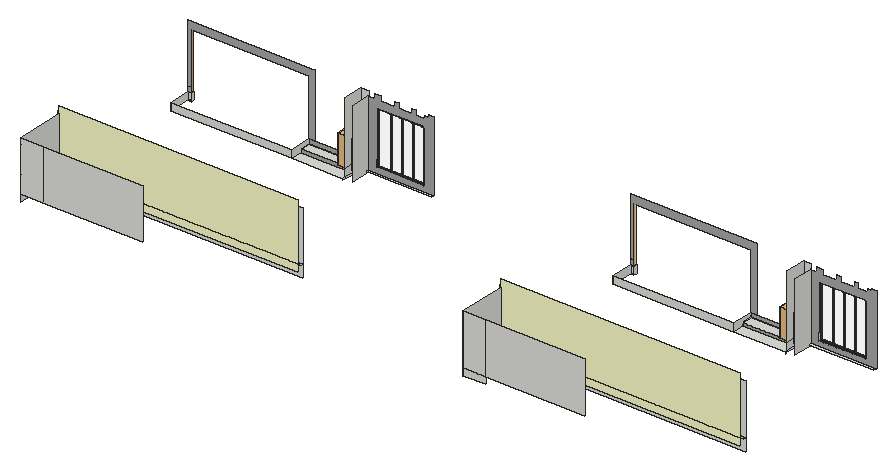
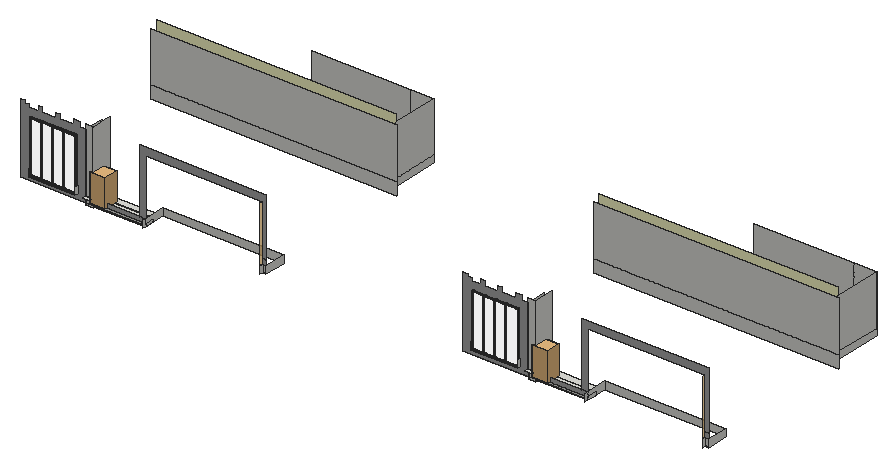
# SketchUp Ruby script. Lengths in inches.
U = 1.inch
M = Sketchup.active_model
def pt(a) = Geom::Point3d.new(a.map { |v| v * U })
def face(e, loops, mat)
  f = e.add_face(loops[0].map { |a| pt(a) })
  loops[1..].each { |l| e.add_face(l.map { |a| pt(a) }).erase! }
  f.material = f.back_material = mat if mat
  f
end
# faces: each face lists its corners as indices into pts; further lists are holes
def faces(e, pts, list, mat = nil) = list.each { |f| face(e, (f[0].is_a?(Array) ? f : [f]).map { |l| l.map { |i| pts[i] } }, mat) }
# xy, xz, yz: faces in a plane at the given z, y or x. An outline is a flat list of corners, or four numbers for a rectangle; further outlines are holes
def ring(l) = l.size == 4 ? [[l[0], l[1]], [l[2], l[1]], [l[2], l[3]], [l[0], l[3]]] : l.each_slice(2).to_a
def flat(e, list, mat, &to3) = list.each { |f| face(e, (f[0].is_a?(Array) ? f : [f]).map { |l| ring(l).map { |u, v| to3.(u, v) } }, mat) }
def xy(e, z, list, mat = nil) = flat(e, list, mat) { |x, y| [x, y, z] }
def xz(e, y, list, mat = nil) = flat(e, list, mat) { |x, z| [x, y, z] }
def yz(e, x, list, mat = nil) = flat(e, list, mat) { |y, z| [x, y, z] }
def lines(e, pts, list) = list.each { |a, b| e.add_line(pt(pts[a]), pt(pts[b])) }
# prism: a flat outline (further loops are holes) pulled along v
def prism(e, loops, v, mat = nil)
  f = face(e, loops, mat); d = Geom::Vector3d.new(v.map { |x| x * U })
  f.pushpull(f.normal.samedirection?(d) ? d.length : -d.length)
end
def box(e, o, s, mat = nil) = prism(e, [[o, [o[0] + s[0], o[1], o[2]], [o[0] + s[0], o[1] + s[1], o[2]], [o[0], o[1] + s[1], o[2]]]], [0, 0, s[2]], mat)
def at(x, y, z, deg = 0) = Geom::Transformation.translation(pt([x, y, z])) * Geom::Transformation.rotation(ORIGIN, Z_AXIS, deg.degrees)
def axes(o, x, y, z) = Geom::Transformation.new([*x, 0, *y, 0, *z, 0, *pt(o).to_a, 1])
def part(name) = M.definitions.add(name)
# library, detail: a bought-in or finely detailed component or shape, given as its bounding box
def library(name, o, s) = part(name).tap { |d| box(d.entities, o, s) }
def detail(e, o, s) = box(e.add_group.entities, o, s)
def put(e, d, t, mat = nil) = e.add_instance(d, t).tap { |i| i.material = mat if mat }
def group(e, t, mat = nil) = e.add_group.tap { |g| g.transformation = t; g.material = mat if mat }.entities
root = M.entities
M.materials.add("Glazing").color = [128, 128, 128]
M.materials["Glazing"].alpha = 0.05
M.materials.add("Powdercoating").color = [41, 44, 40]
M.materials.add("[Color E01]").color = [255, 255, 204]
M.materials.add("[Color M03]1").color = [170, 170, 170]
M.materials.add("[Wood OSB]").color = [255, 207, 129]
M.materials["[Wood OSB]"].alpha = 0.8
c1 = library("plant1",[-367.84,-375.82,-125.45],[750.59,696.16,1346.74])
c2 = part("skp4FF")
put(c2.entities,c1,at(0,0,0))
c3 = part("Group\#15")
xy(c3.entities,0,[[0,-55.94,0.71,45.94]])
xy(c3.entities,0.2,[[0,-55.94,0.47,45.94],[0.47,45.94,0.71,46.42]])
xy(c3.entities,2.36,[[0.47,-55.94,0.71,46.42]])
xz(c3.entities,-55.94,[[0,0,0.71,0,0.71,2.36,0.47,2.36,0.47,0.2,0,0.2]])
xz(c3.entities,45.94,[[0,0,0.71,0.2]])
xz(c3.entities,46.42,[[0.47,0.2,0.71,2.36]])
yz(c3.entities,0,[[-55.94,0,45.94,0.2]])
yz(c3.entities,0.47,[[-55.94,0.2,46.42,2.36]])
yz(c3.entities,0.71,[[-55.94,0,45.94,0,45.94,0.2,46.42,0.2,46.42,2.36,-55.94,2.36]])
c4 = part("Group\#7")
xy(c4.entities,0,[[0,-59.09,0.71,45.94]])
xy(c4.entities,0.2,[[0,-59.09,0.47,45.94],[0.47,45.94,0.71,46.42]])
xy(c4.entities,2.36,[[0.47,-59.09,0.71,46.42]])
xz(c4.entities,-59.09,[[0,0,0.71,0,0.71,2.36,0.47,2.36,0.47,0.2,0,0.2]])
xz(c4.entities,45.94,[[0,0,0.71,0.2]])
xz(c4.entities,46.42,[[0.47,0.2,0.71,2.36]])
yz(c4.entities,0,[[-59.09,0,45.94,0.2]])
yz(c4.entities,0.47,[[-59.09,0.2,46.42,2.36]])
yz(c4.entities,0.71,[[-59.09,0,45.94,0,45.94,0.2,46.42,0.2,46.42,2.36,-59.09,2.36]])
c5 = part("Group\#16")
prism(c5.entities,[[[0.47,-56.18,0.2],[0,-56.18,0.2],[0,-56.18,0],[0.71,-56.18,0],[0.71,-56.18,2.36],[0.47,-56.18,2.36]]],[0,28.68,0])
c6 = part("Group\#10")
box(c6.entities,[-0.73,0,0],[27.99,0.55,102.05])
c7 = part("Group\#18")
xy(c7.entities,0,[[0.47,-56.18,0.47,-55.47,0,-55.47,0,-28.21,1.18,-28.21,1.18,-56.18]])
xy(c7.entities,0.2,[[0.71,-56.18,1.18,-28.21],[0,-55.47,0.47,-28.21],[0.47,-28.21,0.71,-27.74]])
xy(c7.entities,2.36,[[0.47,-56.18,0.71,-27.74]])
xz(c7.entities,-56.18,[[0.47,0,1.18,0,1.18,0.2,0.71,0.2,0.71,2.36,0.47,2.36]])
xz(c7.entities,-55.47,[[0,0,0.47,0.2]])
xz(c7.entities,-28.21,[[0,0,1.18,0.2]])
xz(c7.entities,-27.74,[[0.47,0.2,0.71,2.36]])
yz(c7.entities,0,[[-55.47,0,-28.21,0.2]])
yz(c7.entities,0.47,[[-56.18,0,-55.47,0.2],[-56.18,0.2,-27.74,2.36]])
yz(c7.entities,0.71,[[-56.18,0.2,-27.74,2.36]])
yz(c7.entities,1.18,[[-56.18,0,-28.21,0.2]])
c8 = part("Group\#34")
xy(c8.entities,0,[[-20.45,0,7.76,1.22]])
xy(c8.entities,0.06,[[-20.39,0.06,7.7,1.22]])
xy(c8.entities,0.47,[[-19.98,0,7.28,0.06]])
xy(c8.entities,101.89,[[-19.98,0,7.28,0.06]])
xy(c8.entities,102.3,[[-20.39,0.06,7.7,1.22]])
xy(c8.entities,102.36,[[-20.45,0,7.76,1.22]])
xz(c8.entities,0,[[[-20.45,0,7.76,102.36],[-19.98,0.47,7.28,101.89]]])
xz(c8.entities,0.06,[[[-20.39,0.06,7.7,102.3],[-19.98,0.47,7.28,101.89]]])
xz(c8.entities,1.22,[[[-20.45,0,7.76,102.36],[-20.39,0.06,7.7,102.3]]])
yz(c8.entities,-20.45,[[0,0,1.22,102.36]])
yz(c8.entities,-20.39,[[0.06,0.06,1.22,102.3]])
yz(c8.entities,-19.98,[[0,0.47,0.06,101.89]])
yz(c8.entities,7.28,[[0,0.47,0.06,101.89]])
yz(c8.entities,7.7,[[0.06,0.06,1.22,102.3]])
yz(c8.entities,7.76,[[0,0,1.22,102.36]])
c9 = part("Group\#6")
put(c9.entities,c3,axes([27.97,0,7.875],[1,0,0],[0,0,-1],[0,1,0]),"Powdercoating")
put(c9.entities,c4,axes([0.71,0,6.8],[-1,0,0],[0,0,-0.97687],[0,1,0]),"Powdercoating")
put(c9.entities,c5,axes([-27.5,0,-38.07],[0,0,-1],[-1,0,0],[0,1,0]),"Powdercoating")
put(c9.entities,c6,at(1.12,0.35,-38.39),"Glazing")
put(c9.entities,c7,axes([-27.5,0,63.35],[0,0,1],[-1,0,0],[0,1,0]),"Powdercoating")
put(c9.entities,c8,at(20.6875,1.0625,-38.54),"Powdercoating")
c10 = part("Component\#2")
put(c10.entities,c9,at(-1.18,4.5,38.86))
g1 = group(c10.entities,at(84.74,4.5,38.86))
put(g1,c3,axes([-27.97,0,7.875],[-1,0,0],[0,0,-1],[0,1,0]),"Powdercoating")
put(g1,c4,axes([-0.71,0,6.8],[1,0,0],[0,0,-0.97687],[0,1,0]),"Powdercoating")
put(g1,c5,axes([27.5,0,-38.07],[0,0,-1],[1,0,0],[0,1,0]),"Powdercoating")
put(g1,c6,axes([-1.12,0.35,-38.39],[-1,0,0],[0,1,0],[0,0,1]),"Glazing")
put(g1,c7,axes([27.5,0,63.35],[0,0,1],[1,0,0],[0,1,0]),"Powdercoating")
put(g1,c8,axes([-20.6875,1.0625,-38.54],[-1,0,0],[0,1,0],[0,0,1]),"Powdercoating")
g2 = group(c10.entities,at(56.0625,4.5,38.86))
put(g2,c3,axes([-27.97,0,7.875],[-1,0,0],[0,0,-1],[0,1,0]),"Powdercoating")
put(g2,c5,axes([27.5,0,-38.07],[0,0,-1],[1,0,0],[0,1,0]),"Powdercoating")
put(g2,c6,axes([-1.12,0.35,-38.39],[-1,0,0],[0,1,0],[0,0,1]),"Glazing")
put(g2,c7,axes([27.5,0,63.35],[0,0,1],[1,0,0],[0,1,0]),"Powdercoating")
put(g2,c8,axes([-20.6875,1.0625,-38.54],[-1,0,0],[0,1,0],[0,0,1]),"Powdercoating")
g3 = group(g2,at(-0.71,0,6.8),"Powdercoating")
xy(g3,-45.34,[[0.47,0.2,0.71,2.36]])
xy(g3,-44.88,[[0,0,0.71,0.2]])
xy(g3,57.73,[[0,0,0.71,0,0.71,2.36,0.47,2.36,0.47,0.2,0,0.2]])
xz(g3,0,[[0,-44.88,0.71,57.73]])
xz(g3,0.2,[[0.47,-45.34,0.71,-44.88],[0,-44.88,0.47,57.73]])
xz(g3,2.36,[[0.47,-45.34,0.71,57.73]])
yz(g3,0,[[0,-44.88,0.2,57.73]])
yz(g3,0.47,[[0.2,-45.34,2.36,57.73]])
yz(g3,0.71,[[0.2,-45.34,2.36,-45.34,2.36,57.73,0,57.73,0,-44.88,0.2,-44.88]])
put(c10.entities,c9,axes([-33.94,4.5,38.86],[1.14218,0,0],[0,1,0],[0,0,1]))
c11 = part("sliding door")
put(c11.entities,c10,at(0,-4.5,-0.08))
xy(root,-19.8125,[[486.07,994.94,608.75,1022.06],[1534.38,994.94,1657.0625,1022.06],[486.07,1022.06,608.75,1046.93],[1534.38,1022.06,1657.0625,1046.93]])
xy(root,-18.36,[[626.34,1040.81,782.4375,1046.93],[1674.65,1040.81,1830.75,1046.93]])
xy(root,-12.51,[[486.07,1022.06,608.75,1046.93],[1534.38,1022.06,1657.0625,1046.93]])
xy(root,-5.4375,[[647.11,1046.93,757.11,1054],[1695.43,1046.93,1805.43,1054]])
xy(root,-2.1875,[[608.75,1046.93,626.34,1048.49],[1657.0625,1046.93,1674.65,1048.49],[608.75,1048.49,626.34,1057.1875],[1657.0625,1048.49,1674.65,1057.1875]])
xz(root,538.16,[[1257.22,-9.875,1311.1,6.75],[208.91,6.75,262.79,126.75],[262.79,6.75,499.53,126.75],[1257.22,6.75,1311.1,126.75],[1311.1,6.75,1547.84,126.75]])
xz(root,652.02,[[208.91,-9.875,775.16,6.75],[1257.22,-9.875,1823.47,6.75],[208.91,6.75,775.16,144.3125],[1257.22,6.75,1823.47,144.3125]],"[Color E01]")
xz(root,659.09,[[200.03,-22.8,782.78,6.75],[1248.34,-22.8,1831.09,6.75],[200.03,6.75,782.78,126.75],[1248.34,6.75,1831.09,126.75]])
xz(root,994.94,[[199.6875,-19.8125,486.07,-2.1875],[1248,-19.8125,1534.38,-2.1875]])
xz(root,1022.06,[[486.07,-19.8125,608.75,-12.51],[1534.38,-19.8125,1657.0625,-12.51]],"[Color M03]1")
xz(root,1046.93,[[608.75,-23.22,626.34,-18.36],[1657.0625,-23.22,1674.65,-18.36],[199.6875,-19.8125,208.57,-18.36],[486.07,-19.8125,608.75,-18.36],[1248,-19.8125,1256.88,-18.36],
  [1534.38,-19.8125,1657.0625,-18.36],[199.6875,-18.36,208.57,-2.1875],[486.07,-18.36,608.75,-12.51],[608.75,-18.36,626.34,-2.1875],[1248,-18.36,1256.88,-2.1875],
  [1534.38,-18.36,1657.0625,-12.51],[1657.0625,-18.36,1674.65,-2.1875]])
xz(root,1046.93,[[[626.34,-18.36,782.4375,-18.36,782.4375,148.75,771.14,148.75,771.14,143.9375,761.39,143.9375,761.39,138.0625,738.93,138.0625,738.93,148.75,730.52,148.75,730.52,138.0625,698.31,138.0625,698.31,148.75,688.89,148.75,688.89,138.0625,656.68,138.0625,656.68,148.75,641.2,148.75,641.2,138.0625,626.34,138.0625],[647.11,-5.4375,757.11,120.25]],[[1674.65,-18.36,1830.75,-18.36,1830.75,148.75,1819.45,148.75,1819.45,143.9375,1809.71,143.9375,1809.71,138.0625,1787.25,138.0625,1787.25,148.75,1778.83,148.75,1778.83,138.0625,1746.62,138.0625,1746.62,148.75,1737.2,148.75,1737.2,138.0625,1705,138.0625,1705,148.75,1689.52,148.75,1689.52,138.0625,1674.65,138.0625],[1695.43,-5.4375,1805.43,120.25]],[486.07,-12.51,608.75,-2.1875],[1534.38,-12.51,1657.0625,-2.1875],[199.6875,-2.1875,208.57,11.1875],
  [486.07,-2.1875,499.1875,-2.1875,499.1875,148.75,497.26,148.75,497.26,149.375,199.6875,149.375,199.6875,11.1875,208.57,11.1875,208.57,131.1875,486.07,131.1875],[1248,-2.1875,1256.88,11.1875],[1534.38,-2.1875,1547.5,-2.1875,1547.5,148.75,1545.57,148.75,1545.57,149.375,1248,149.375,1248,11.1875,1256.88,11.1875,1256.88,131.1875,1534.38,131.1875]],"[Color M03]1")
xz(root,1048.49,[[608.75,-2.1875,626.34,149.375],[1657.0625,-2.1875,1674.65,149.375]])
yz(root,199.6875,[[994.94,-19.8125,1046.93,-2.1875]])
yz(root,208.57,[[1046.93,-19.8125,1054,-2.1875]])
yz(root,208.57,[[1046.93,-2.1875,1054,131.1875]],"[Wood OSB]")
yz(root,208.91,[[538.16,-9.875,652.02,6.75],[538.16,6.75,652.02,126.75]])
yz(root,486.07,[[994.94,-19.8125,1022.06,-19.8125,1022.06,-12.51,1046.93,-12.51,1046.93,-2.1875,994.94,-2.1875],[1022.06,-19.8125,1023.55,-19.8125,1023.55,-12.51,1022.06,-13.17],[1023.55,-19.8125,1046.93,-12.51],[1046.93,-19.8125,1054,-2.1875],[1022.06,-13.17,1023.55,-12.51,1022.06,-12.51]])
yz(root,608.75,[[994.94,-23.22,1000.12,-19.8125],[1000.12,-23.22,1022.06,-19.8125],[1022.06,-23.22,1046.93,-19.8125],[1000.12,-19.8125,1000.12,-2.1875,1046.93,-2.1875,1046.93,-12.51,1022.06,-12.51,1022.06,-19.8125],[1022.06,-19.8125,1046.93,-12.51],
  [1000.12,-2.1875,1000.12,149.375,1024.56,149.375,1024.56,148.75,1048.49,148.75,1048.49,-2.1875]])
yz(root,626.34,[[1000.12,-23.22,1040.81,-23.22,1040.81,-18.36,1046.93,-18.36,1046.93,138.0625,1000.12,138.0625],[1040.81,-23.22,1046.93,-18.36],[1046.93,-2.1875,1048.49,138.0625]])
yz(root,647.11,[[1046.93,-5.4375,1054,11.1875]])
yz(root,757.11,[[1046.93,-5.4375,1054,11.1875]])
yz(root,1248,[[994.94,-19.8125,1046.93,-2.1875]])
yz(root,1256.88,[[1046.93,-19.8125,1054,-2.1875]])
yz(root,1256.88,[[1046.93,-2.1875,1054,131.1875]],"[Wood OSB]")
yz(root,1257.22,[[538.16,-9.875,652.02,6.75],[538.16,6.75,652.02,126.75]])
yz(root,1534.38,[[994.94,-19.8125,1022.06,-19.8125,1022.06,-12.51,1046.93,-12.51,1046.93,-2.1875,994.94,-2.1875],[1022.06,-19.8125,1023.55,-19.8125,1023.55,-12.51,1022.06,-13.17],[1023.55,-19.8125,1046.93,-12.51],[1046.93,-19.8125,1054,-2.1875],[1022.06,-13.17,1023.55,-12.51,1022.06,-12.51]])
yz(root,1657.0625,[[994.94,-23.22,1000.12,-19.8125],[1000.12,-23.22,1022.06,-19.8125],[1022.06,-23.22,1046.93,-19.8125],[1000.12,-19.8125,1000.12,-2.1875,1046.93,-2.1875,1046.93,-12.51,1022.06,-12.51,1022.06,-19.8125],[1022.06,-19.8125,1046.93,-12.51],
  [1000.12,-2.1875,1000.12,149.375,1024.56,149.375,1024.56,148.75,1048.49,148.75,1048.49,-2.1875]])
yz(root,1674.65,[[1000.12,-23.22,1040.81,-23.22,1040.81,-18.36,1046.93,-18.36,1046.93,138.0625,1000.12,138.0625],[1040.81,-23.22,1046.93,-18.36],[1046.93,-2.1875,1048.49,138.0625]])
yz(root,1695.43,[[1046.93,-5.4375,1054,11.1875]])
yz(root,1805.43,[[1046.93,-5.4375,1054,11.1875]])
p = [[782.78,652.02,6.75],[775.16,652.02,6.75],[782.78,659.09,6.75],[1831.09,652.02,6.75],[1823.47,652.02,6.75],[1831.09,659.09,6.75]]
lines(root,p,[[0,1],[0,2],[3,4],[3,5]])
put(root,c2,axes([594.89,1036.62,-5.66],[0.04953,0,0],[0,0.04953,0],[0,0,0.04953]))
put(root,c2,axes([1643.2,1036.62,-5.66],[0.04953,0,0],[0,0.04953,0],[0,0,0.04953]))
put(root,c11,axes([679.9,1048.71,-5.4375],[0.91114,0,0],[0,0.755,0],[0,0,1.2092]))
put(root,c11,axes([1728.21,1048.71,-5.4375],[0.91114,0,0],[0,0.755,0],[0,0,1.2092]))
